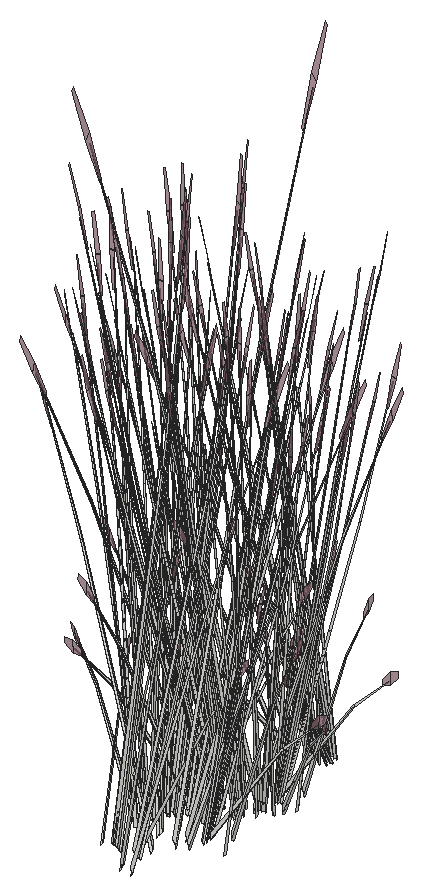
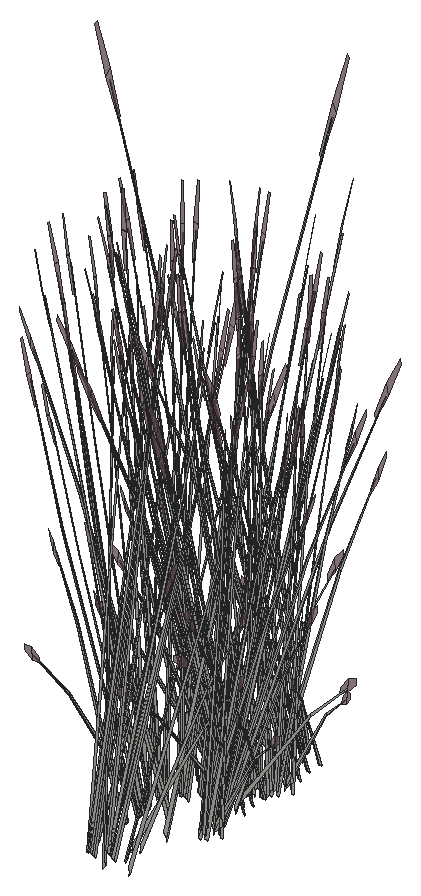
# SketchUp Ruby script. Lengths in inches.
U = 1.inch
M = Sketchup.active_model
def pt(a) = Geom::Point3d.new(a.map { |v| v * U })
def face(e, loops, mat)
  f = e.add_face(loops[0].map { |a| pt(a) })
  loops[1..].each { |l| e.add_face(l.map { |a| pt(a) }).erase! }
  f.material = f.back_material = mat if mat
  f
end
# faces: each face lists its corners as indices into pts; further lists are holes
def faces(e, pts, list, mat = nil) = list.each { |f| face(e, (f[0].is_a?(Array) ? f : [f]).map { |l| l.map { |i| pts[i] } }, mat) }
# xy, xz, yz: faces in a plane at the given z, y or x. An outline is a flat list of corners, or four numbers for a rectangle; further outlines are holes
def ring(l) = l.size == 4 ? [[l[0], l[1]], [l[2], l[1]], [l[2], l[3]], [l[0], l[3]]] : l.each_slice(2).to_a
def flat(e, list, mat, &to3) = list.each { |f| face(e, (f[0].is_a?(Array) ? f : [f]).map { |l| ring(l).map { |u, v| to3.(u, v) } }, mat) }
def xy(e, z, list, mat = nil) = flat(e, list, mat) { |x, y| [x, y, z] }
def xz(e, y, list, mat = nil) = flat(e, list, mat) { |x, z| [x, y, z] }
def yz(e, x, list, mat = nil) = flat(e, list, mat) { |y, z| [x, y, z] }
def lines(e, pts, list) = list.each { |a, b| e.add_line(pt(pts[a]), pt(pts[b])) }
# prism: a flat outline (further loops are holes) pulled along v
def prism(e, loops, v, mat = nil)
  f = face(e, loops, mat); d = Geom::Vector3d.new(v.map { |x| x * U })
  f.pushpull(f.normal.samedirection?(d) ? d.length : -d.length)
end
def box(e, o, s, mat = nil) = prism(e, [[o, [o[0] + s[0], o[1], o[2]], [o[0] + s[0], o[1] + s[1], o[2]], [o[0], o[1] + s[1], o[2]]]], [0, 0, s[2]], mat)
def at(x, y, z, deg = 0) = Geom::Transformation.translation(pt([x, y, z])) * Geom::Transformation.rotation(ORIGIN, Z_AXIS, deg.degrees)
def axes(o, x, y, z) = Geom::Transformation.new([*x, 0, *y, 0, *z, 0, *pt(o).to_a, 1])
def part(name) = M.definitions.add(name)
# library, detail: a bought-in or finely detailed component or shape, given as its bounding box
def library(name, o, s) = part(name).tap { |d| box(d.entities, o, s) }
def detail(e, o, s) = box(e.add_group.entities, o, s)
def put(e, d, t, mat = nil) = e.add_instance(d, t).tap { |i| i.material = mat if mat }
def group(e, t, mat = nil) = e.add_group.tap { |g| g.transformation = t; g.material = mat if mat }.entities
root = M.entities
M.materials.add("LightPink_Translucent").color = [144, 107, 117]
M.materials["LightPink_Translucent"].alpha = 0.75
c1 = part("blade")
p = [[2.15,0.21,22],[0,0.17,0],[0.09,0.45,0],[2.18,0.31,22],[2.29,0.31,22],[0.38,0.45,0],
  [2.48,0.24,33],[2.49,0.24,33],[2.48,0.22,33]]
faces(c1.entities,p,[[0,1,2,3],[4,5,2,3],[6,3,4,7],[8,0,3,6]])
c2 = part("seeds")
p = [[0.3,-0.1,1.38],[-0.01,-0.03,1.59],[-0.01,-0.03,0.03],[0.14,-0.07,-0.07],[0.29,-0.03,3],[0.15,0.01,3.11]]
faces(c2.entities,p,[[0,1,2,3],[1,0,4,5]],"LightPink_Translucent")
c3 = part("blade with seeds")
put(c3.entities,c1,at(0,0,0))
put(c3.entities,c2,axes([2.4,0.25,30.99],[1.5799,-0.05474,1.17369],[-0.12525,1.92788,0.29478],[-0.07173,-0.02425,1.56792]))
put(root,c3,axes([426.9,471.09,153.98],[-0.01019,0.09334,1.47793],[0.28908,0.3247,-0.23373],[-0.07568,0.15355,0.11853]))
put(root,c3,axes([427.82,470.88,154.56],[0.45039,0.02337,-0.11403],[-0.01231,0.44247,-0.63292],[-0.03129,0.17041,0.9617]))
put(root,c3,axes([428.66,471.37,154.25],[0.40102,-0.2196,-0.10273],[0.19707,0.38974,-0.57019],[0.05291,0.16424,0.8664]))
put(root,c3,axes([431.05,474.26,154],[0.15051,0.3216,0.05432],[-0.27447,0.15741,0.42765],[0.12099,-0.03106,0.65209]))
put(root,c3,axes([429.21,477.45,153.95],[-0.40284,-0.11824,-0.43168],[0.13808,-0.40538,-0.33437],[-0.03694,-0.16321,0.82598]))
put(root,c3,axes([431.03,474.15,154],[-0.11578,0.43006,0.40553],[-0.38064,-0.14706,0.33437],[0.14969,-0.02584,0.83914]))
put(root,c3,axes([430.08,477.75,153.95],[-0.29336,-0.31691,-0.43168],[0.3099,-0.27755,-0.33437],[0.04464,-0.16102,0.82598]))
put(root,c3,axes([428.49,476.19,153.98],[-0.00765,0.05653,1.49853],[-0.37706,0.20517,-0.1416],[-0.11096,-0.10488,0.26519]))
put(root,c3,axes([428.13,471.05,154.23],[0.29336,0.31691,-0.47917],[-0.3099,0.27755,-0.37115],[-0.04464,0.16102,0.91684]))
put(root,c3,axes([429,471.35,153.95],[0.40284,0.11824,-0.43168],[-0.13808,0.40538,-0.33437],[0.03694,0.16321,0.82598]))
put(root,c3,axes([428.14,473.42,152.82],[0.11649,-0.06823,1.49584],[0.04017,0.47639,0.11706],[-0.25231,0.06321,0.53462]))
put(root,c3,axes([429.23,470.52,153.27],[-0.09368,-0.15143,1.44779],[0.43286,-0.12749,0.11706],[0.09783,0.23774,0.61892]))
put(root,c3,axes([429.43,477.28,154],[0.4038,0.12331,0.40553],[-0.13808,0.40538,0.33437],[-0.02427,-0.15942,0.83914]))
put(root,c3,axes([429.55,477.43,154.25],[-0.40102,0.2196,-0.10273],[-0.19707,-0.38974,-0.57019],[-0.05291,-0.16424,0.8664]))
put(root,c3,axes([430.38,477.92,154.25],[-0.45039,-0.02337,-0.10273],[0.01231,-0.44247,-0.57019],[0.03129,-0.17041,0.8664]))
put(root,c3,axes([430.35,477.64,153.82],[0.27728,-0.24833,-0.29918],[0.26248,0.28355,0.38624],[0.03994,-0.14407,0.73904]))
put(root,c3,axes([428.82,471.6,153.82],[-0.12355,0.36271,-0.29918],[-0.36044,-0.10579,0.38624],[0.03305,0.14603,0.73904]))
put(root,c3,axes([429.54,477.25,154],[0.30197,-0.1603,0.05432],[0.1478,0.29231,0.42765],[-0.02916,-0.12885,0.65209]))
put(root,c3,axes([428.35,477.33,153.82],[-0.06329,-0.37991,-0.29918],[0.36182,-0.10032,0.38624],[-0.09718,-0.10887,0.73904]))
put(root,c3,axes([428.04,470.9,154.51],[-0.01066,0.43628,-0.66621],[-0.44902,-0.0293,0.0804],[-0.04739,0.18483,0.94242]))
put(root,c3,axes([431.71,475.54,153.98],[-0.03706,-0.04129,1.49853],[0.08106,-0.44261,-0.1416],[0.14596,-0.02828,0.26519]))
put(root,c3,axes([426.87,472.05,153.98],[0.04649,-0.02848,1.49853],[0.38427,0.18941,-0.1416],[-0.00903,0.15771,0.26519]))
put(root,c3,axes([426.89,473.74,153.98],[-0.06692,0.06124,1.47793],[0.00569,0.44742,-0.23373],[-0.15339,0.05818,0.11853]))
put(root,c3,axes([427.34,473.68,153.95],[-0.11102,0.42903,-0.43168],[-0.38064,-0.14706,-0.33437],[-0.15325,0.03934,0.82598]))
put(root,c3,axes([427.32,473.32,154.25],[0.20619,0.42709,-0.10273],[-0.36595,0.20988,-0.57019],[-0.15422,0.05635,0.8664]))
put(root,c3,axes([428.46,470.59,153.27],[-0.01003,-0.18103,1.44779],[0.43473,0.12009,0.11706],[-0.02689,0.25798,0.61892]))
put(root,c3,axes([431.39,475.17,153.32],[-0.07843,-0.39649,-0.0295],[0.37072,-0.09115,-0.13375],[0.07742,0.02514,0.44114]))
put(root,c3,axes([430.43,475.16,154.25],[0.02194,-0.47967,-0.10273],[0.41546,0.01311,-0.57019],[0.16001,0.03332,0.8664]))
put(root,c3,axes([428.51,477.3,154],[0.18625,-0.29962,0.05432],[0.26523,0.17444,0.42765],[-0.08575,-0.09606,0.65209]))
put(root,c3,axes([427.57,477.88,153.27],[0.15222,0.08126,1.44779],[-0.31502,0.34091,0.11706],[-0.19634,-0.15379,0.61892]))
put(root,c3,axes([428.5625,472.24,153.98],[0.05195,0.07595,1.47793],[0.41921,0.02984,-0.23373],[0.04216,0.1675,0.11853]))
put(root,c3,axes([428.31,477.64,153.95],[-0.40438,0.11212,-0.43168],[-0.07074,-0.4246,-0.33437],[-0.10862,-0.12168,0.82598]))
put(root,c3,axes([430.35,477.73,154],[0.29182,0.32181,0.40553],[-0.3099,0.27755,0.33437],[0.05383,-0.15098,0.83914]))
put(root,c3,axes([428.59,477.27,154.59],[-0.2735,0.45217,-0.11506],[-0.39608,-0.2605,-0.63862],[-0.13768,-0.12775,0.97037]))
put(root,c3,axes([430.46,477.76,154],[0.33677,0.02198,0.05432],[-0.00923,0.33185,0.42765],[0.03524,-0.12712,0.65209]))
put(root,c3,axes([430.79,474.87,153.98],[0.08791,-0.00798,1.47793],[0.24113,-0.36643,-0.23373],[0.15637,0.04837,0.11853]))
put(root,c3,axes([427.27,474.51,154],[-0.10163,-0.43409,0.40553],[0.39868,-0.07534,0.33437],[-0.1175,0.10209,0.83914]))
put(root,c3,axes([427.19,474.43,154],[-0.28133,-0.19836,0.05432],[0.16379,-0.28248,0.42765],[-0.0902,0.09132,0.65209]))
put(root,c3,axes([427.32,473.91,153.27],[0.14219,-0.09977,1.44779],[0.11971,0.461,0.11706],[-0.22323,0.10419,0.61892]))
put(root,c3,axes([430.6875,478.48,153.95],[-0.10528,-0.43067,-0.43168],[0.39868,-0.07534,-0.33437],[0.11425,-0.11568,0.82598]))
put(root,c3,axes([427.89,471.51,152.84],[0.009,-0.24349,1.30391],[0.40497,0.12861,0.18019],[-0.03509,0.2595,0.61571]))
put(root,c3,axes([427.54,477.14,153.98],[-0.08817,-0.00333,1.47793],[-0.28072,0.33293,-0.23373],[-0.14978,-0.06803,0.11853]))
put(root,c3,axes([430.875,478.79,154.25],[-0.37908,-0.26007,-0.10273],[0.21839,-0.37663,-0.57019],[0.1071,-0.13092,0.8664]))
put(root,c3,axes([429.31,480.21,152.81],[0.35414,0.19019,1.27785],[-0.34693,0.40974,0.50532],[-0.1554,-0.24285,1.07126]))
put(root,c3,axes([426.14,474.2,153.98],[0.0523,0.01265,1.49853],[0.16179,0.41674,-0.1416],[-0.10706,0.10938,0.26519]))
put(root,c3,axes([431.81,478.68,153.98],[-0.05353,-0.00358,1.49853],[-0.22227,-0.38383,-0.1416],[0.08926,-0.1262,0.26519]))
put(root,c3,axes([430.69,475.125,153.82],[0.23317,0.29531,-0.29918],[-0.26625,0.27955,0.38624],[0.13527,0.04253,0.73904]))
put(root,c3,axes([430.57,475.24,154],[-0.02064,0.35866,0.05432],[-0.3116,-0.00983,0.42765],[0.11936,0.03753,0.65209]))
put(root,c3,axes([427.23,474.6,153.82],[-0.35672,0.06741,-0.29918],[-0.09419,-0.38534,0.38624],[-0.10222,0.1035,0.73904]))
put(root,c3,axes([430.6,475.125,154],[-0.30217,0.31079,0.40553],[-0.2606,-0.33005,0.33437],[0.14177,0.05733,0.83914]))
put(root,c3,axes([430.98,478.53,153.82],[0.35672,-0.06741,-0.29918],[0.09419,0.38534,0.38624],[0.10222,-0.1035,0.73904]))
put(root,c3,axes([427.63,477.89,154],[0.02064,-0.35866,0.05432],[0.3116,0.00983,0.42765],[-0.11936,-0.03753,0.65209]))
put(root,c3,axes([427.51,478,153.82],[-0.23317,-0.29531,-0.29918],[0.26625,-0.27955,0.38624],[-0.13527,-0.04253,0.73904]))
put(root,c3,axes([429.86,474.37,153.27],[-0.15222,-0.08126,1.44779],[0.31502,-0.34091,0.11706],[0.19634,0.15379,0.61892]))
put(root,c3,axes([429.88,473.3,153.78],[-0.35411,-0.24507,1.16821],[0.37391,-0.38156,0.50405],[0.11425,0.22994,1.12919]))
put(root,c3,axes([427.33,474.33,154.25],[0.37908,0.26007,-0.10273],[-0.21839,0.37663,-0.57019],[-0.1071,0.13092,0.8664]))
put(root,c3,axes([429.61,475.68,154.25],[0.2442,-0.40372,-0.10273],[0.35364,0.23259,-0.57019],[0.12293,0.11406,0.8664]))
put(root,c3,axes([427.84,474.22,153.27],[0.10236,-0.14492,1.44779],[0.25844,0.39118,0.11706],[-0.17726,0.17814,0.61892]))
put(root,c3,axes([427.52,474.64,153.95],[0.10528,0.43067,-0.43168],[-0.39868,0.07534,-0.33437],[-0.11425,0.11568,0.82598]))
put(root,c3,axes([431.01,478.7,154],[0.28133,0.19836,0.05432],[-0.16379,0.28248,0.42765],[0.0902,-0.09132,0.65209]))
put(root,c3,axes([430.93,478.61,154],[0.10163,0.43409,0.40553],[-0.39868,0.07534,0.33437],[0.1175,-0.10209,0.83914]))
put(root,c3,axes([432.01,479.14,153.98],[0.05687,-0.07184,1.47793],[-0.07279,-0.44069,-0.23373],[0.14268,-0.08356,0.11853]))
put(root,c3,axes([429.29,476.02,153.98],[0.00121,-0.0571,1.49853],[0.35119,-0.25193,-0.1416],[0.12199,0.08992,0.26519]))
put(root,c3,axes([427.75,475.36,154],[-0.33677,-0.02198,0.05432],[0.00923,-0.33185,0.42765],[-0.03524,0.12712,0.65209]))
put(root,c3,axes([427.85,475.39,154],[-0.29182,-0.32181,0.40553],[0.3099,-0.27755,0.33437],[-0.05383,0.15098,0.83914]))
put(root,c3,axes([429.9,475.48,153.95],[0.40438,-0.11212,-0.43168],[0.07074,0.4246,-0.33437],[0.10862,0.12168,0.82598]))
put(root,c3,axes([427.2,477.42,153.98],[0.03038,0.04707,1.49853],[-0.14646,0.42312,-0.1416],[-0.14833,0.00306,0.26519]))
put(root,c3,axes([427.625,478.29,153.95],[-0.29757,0.31243,-0.43168],[-0.2606,-0.33005,-0.33437],[-0.15119,-0.04754,0.82598]))
put(root,c3,axes([429.7,475.83,154],[-0.18625,0.29962,0.05432],[-0.26523,-0.17444,0.42765],[0.08575,0.09606,0.65209]))
put(root,c3,axes([427.78,477.97,154.25],[-0.02194,0.47967,-0.10273],[-0.41546,-0.01311,-0.57019],[-0.16001,-0.03332,0.8664]))
put(root,c3,axes([429.78,475.74,154],[-0.4076,0.10824,0.40553],[-0.07074,-0.4246,0.33437],[0.09586,0.12514,0.83914]))
put(root,c3,axes([430.89,479.81,154.25],[-0.20619,-0.42709,-0.10273],[0.36595,-0.20988,-0.57019],[0.15422,-0.05635,0.8664]))
put(root,c3,axes([430.87,479.44,153.95],[0.11102,-0.42903,-0.43168],[0.38064,0.14706,-0.33437],[0.15325,-0.03934,0.82598]))
put(root,c3,axes([427.25,478.63,153.27],[0.16998,-0.01068,1.44779],[-0.11276,0.46299,0.11706],[-0.24224,-0.02864,0.61892]))
put(root,c3,axes([427.77,474.57,153.27],[0.0763,-0.16212,1.44779],[0.3201,0.3355,0.11706],[-0.1444,0.2091,0.61892]))
put(root,c3,axes([428.66,475.87,154],[-0.30197,0.1603,0.05432],[-0.1478,-0.29231,0.42765],[0.02916,0.12885,0.65209]))
put(root,c3,axes([427.85,475.49,153.82],[-0.27728,0.24833,-0.29918],[-0.26248,-0.28355,0.38624],[-0.03994,0.14407,0.73904]))
put(root,c3,axes([426.9,475.41,153.98],[-0.01019,0.09334,1.47793],[0.28908,0.3247,-0.23373],[-0.07568,0.15355,0.11853]))
put(root,c3,axes([427.82,475.2,154.56],[0.45039,0.02337,-0.11403],[-0.01231,0.44247,-0.63292],[-0.03129,0.17041,0.9617]))
put(root,c3,axes([428.66,475.7,154.25],[0.40102,-0.2196,-0.10273],[0.19707,0.38974,-0.57019],[0.05291,0.16424,0.8664]))
put(root,c3,axes([428.13,475.37,154.23],[0.29336,0.31691,-0.47917],[-0.3099,0.27755,-0.37115],[-0.04464,0.16102,0.91684]))
put(root,c3,axes([427.18,478.98,154],[0.11578,-0.43006,0.40553],[0.38064,0.14706,0.33437],[-0.14969,0.02584,0.83914]))
put(root,c3,axes([429,475.68,153.95],[0.40284,0.11824,-0.43168],[-0.13808,0.40538,-0.33437],[0.03694,0.16321,0.82598]))
put(root,c3,axes([429.23,474.84,153.27],[-0.09368,-0.15143,1.44779],[0.43286,-0.12749,0.11706],[0.09783,0.23774,0.61892]))
put(root,c3,axes([427.15,478.86,154],[-0.15051,-0.3216,0.05432],[0.27447,-0.15741,0.42765],[-0.12099,0.03106,0.65209]))
put(root,c3,axes([428.82,475.93,153.82],[-0.12355,0.36271,-0.29918],[-0.36044,-0.10579,0.38624],[0.03305,0.14603,0.73904]))
put(root,c3,axes([428.04,475.23,154.51],[-0.01066,0.43628,-0.66621],[-0.44902,-0.0293,0.0804],[-0.04739,0.18483,0.94242]))
put(root,c3,axes([426.87,476.37,153.98],[0.04649,-0.02848,1.49853],[0.38427,0.18941,-0.1416],[-0.00903,0.15771,0.26519]))
put(root,c3,axes([431.1,479.64,153.82],[0.34057,0.13158,-0.29918],[-0.09933,0.38387,0.38624],[0.13712,-0.0352,0.73904]))
put(root,c3,axes([428.46,474.92,153.27],[-0.01003,-0.18103,1.44779],[0.43473,0.12009,0.11706],[-0.02689,0.25798,0.61892]))
put(root,c3,axes([427.1,479.02,153.82],[-0.34057,-0.13158,-0.29918],[0.09933,-0.38387,0.38624],[-0.13712,0.0352,0.73904]))
put(root,c3,axes([430.18,479.16,153.27],[-0.16998,0.01068,1.44779],[0.11276,-0.46299,0.11706],[0.24224,0.02864,0.61892]))
put(root,c3,axes([428.5625,476.57,153.98],[0.05195,0.07595,1.47793],[0.41921,0.02984,-0.23373],[0.04216,0.1675,0.11853]))
put(root,c3,axes([431.05,479.8,154],[0.15051,0.3216,0.05432],[-0.27447,0.15741,0.42765],[0.12099,-0.03106,0.65209]))
put(root,c3,axes([431.03,479.68,154],[-0.11578,0.43006,0.40553],[-0.38064,-0.14706,0.33437],[0.14969,-0.02584,0.83914]))
put(root,c3,axes([428.14,478.96,152.82],[0.11649,-0.06823,1.49584],[0.04017,0.47639,0.11706],[-0.25231,0.06321,0.53462]))
put(root,c3,axes([427.89,475.84,152.84],[0.009,-0.24349,1.30391],[0.40497,0.12861,0.18019],[-0.03509,0.2595,0.61571]))
put(root,c3,axes([431.71,481.08,153.98],[-0.03706,-0.04129,1.49853],[0.08106,-0.44261,-0.1416],[0.14596,-0.02828,0.26519]))
put(root,c3,axes([426.89,479.28,153.98],[-0.06692,0.06124,1.47793],[0.00569,0.44742,-0.23373],[-0.15339,0.05818,0.11853]))
put(root,c3,axes([427.34,479.22,153.95],[-0.11102,0.42903,-0.43168],[-0.38064,-0.14706,-0.33437],[-0.15325,0.03934,0.82598]))
put(root,c3,axes([427.32,478.85,154.25],[0.20619,0.42709,-0.10273],[-0.36595,0.20988,-0.57019],[-0.15422,0.05635,0.8664]))
put(root,c3,axes([428.2,484.625,153.27],[0.09368,0.15143,1.44779],[-0.43286,0.12749,0.11706],[-0.09783,-0.23774,0.61892]))
put(root,c3,axes([431.39,480.71,153.32],[-0.07843,-0.39649,-0.0295],[0.37072,-0.09115,-0.13375],[0.07742,0.02514,0.44114]))
put(root,c3,axes([430.43,480.69,154.25],[0.02194,-0.47967,-0.10273],[0.41546,0.01311,-0.57019],[0.16001,0.03332,0.8664]))
put(root,c3,axes([428.91,483.62,153.98],[-0.06268,-0.06613,1.47793],[-0.4183,0.04193,-0.23373],[-0.06676,-0.15817,0.11853]))
put(root,c3,axes([429.35,484.74,154.21],[-0.19559,-0.38351,-0.60019],[0.40262,-0.21373,0.07243],[-0.04574,-0.1853,0.84903]))
put(root,c3,axes([430.17,485.11,154.21],[0.01066,-0.43628,-0.60019],[0.44902,0.0293,0.07243],[0.04739,-0.18483,0.84903]))
put(root,c3,axes([430.79,480.41,153.98],[0.08791,-0.00798,1.47793],[0.24113,-0.36643,-0.23373],[0.15637,0.04837,0.11853]))
put(root,c3,axes([427.27,480.05,154],[-0.10163,-0.43409,0.40553],[0.39868,-0.07534,0.33437],[-0.1175,0.10209,0.83914]))
put(root,c3,axes([430.79,484.43,153.98],[-0.00396,-0.09387,1.47793],[-0.33411,-0.2713,-0.23373],[0.05166,-0.16446,0.11853]))
put(root,c3,axes([429.39,484.41,153.82],[0.12355,-0.36271,-0.29918],[0.36044,0.10579,0.38624],[-0.03305,-0.14603,0.73904]))
put(root,c3,axes([429.66,484.89,153.27],[-0.0763,0.16212,1.44779],[-0.3201,-0.3355,0.11706],[0.1444,-0.2091,0.61892]))
put(root,c3,axes([427.19,479.96,154],[-0.28133,-0.19836,0.05432],[0.16379,-0.28248,0.42765],[-0.0902,0.09132,0.65209]))
put(root,c3,axes([430.7,484.09,153.98],[-0.04162,0.03603,1.49853],[-0.40776,-0.12155,-0.1416],[-0.01476,-0.15722,0.26519]))
put(root,c3,axes([427.32,479.44,153.27],[0.14219,-0.09977,1.44779],[0.11971,0.461,0.11706],[-0.22323,0.10419,0.61892]))
put(root,c3,axes([429.21,484.66,153.95],[-0.40284,-0.11824,-0.43168],[0.13808,-0.40538,-0.33437],[-0.03694,-0.16321,0.82598]))
put(root,c3,axes([430.08,484.97,153.95],[-0.29336,-0.31691,-0.43168],[0.3099,-0.27755,-0.33437],[0.04464,-0.16102,0.82598]))
put(root,c3,axes([428.49,483.4,153.98],[-0.00765,0.05653,1.49853],[-0.37706,0.20517,-0.1416],[-0.11096,-0.10488,0.26519]))
put(root,c3,axes([426.14,479.73,153.98],[0.0523,0.01265,1.49853],[0.16179,0.41674,-0.1416],[-0.10706,0.10938,0.26519]))
put(root,c3,axes([429.43,484.5,154],[0.4038,0.12331,0.40553],[-0.13808,0.40538,0.33437],[-0.02427,-0.15942,0.83914]))
put(root,c3,axes([429.55,484.64,154.25],[-0.40102,0.2196,-0.10273],[-0.19707,-0.38974,-0.57019],[-0.05291,-0.16424,0.8664]))
put(root,c3,axes([430.69,480.66,153.82],[0.23317,0.29531,-0.29918],[-0.26625,0.27955,0.38624],[0.13527,0.04253,0.73904]))
put(root,c3,axes([430.38,485.13,154.25],[-0.45039,-0.02337,-0.10273],[0.01231,-0.44247,-0.57019],[0.03129,-0.17041,0.8664]))
put(root,c3,axes([430.35,484.85,153.82],[0.27728,-0.24833,-0.29918],[0.26248,0.28355,0.38624],[0.03994,-0.14407,0.73904]))
put(root,c3,axes([429.54,484.47,154],[0.30197,-0.1603,0.05432],[0.1478,0.29231,0.42765],[-0.02916,-0.12885,0.65209]))
put(root,c3,axes([430.57,480.77,154],[-0.02064,0.35866,0.05432],[-0.3116,-0.00983,0.42765],[0.11936,0.03753,0.65209]))
put(root,c3,axes([428.35,484.55,153.82],[-0.06329,-0.37991,-0.29918],[0.36182,-0.10032,0.38624],[-0.09718,-0.10887,0.73904]))
put(root,c3,axes([427.23,480.13,153.82],[-0.35672,0.06741,-0.29918],[-0.09419,-0.38534,0.38624],[-0.10222,0.1035,0.73904]))
put(root,c3,axes([430.6,480.66,154],[-0.30217,0.31079,0.40553],[-0.2606,-0.33005,0.33437],[0.14177,0.05733,0.83914]))
